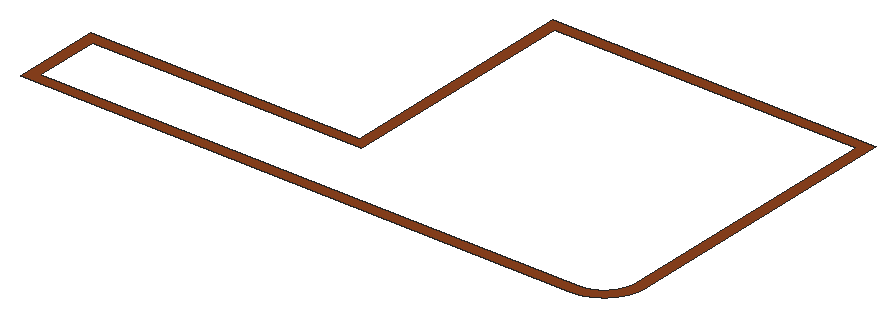
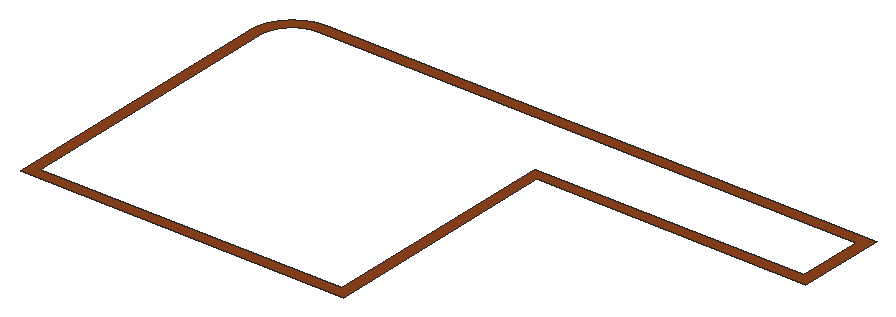
# SketchUp Ruby script. Lengths in inches.
U = 1.inch
M = Sketchup.active_model
def pt(a) = Geom::Point3d.new(a.map { |v| v * U })
def face(e, loops, mat)
  f = e.add_face(loops[0].map { |a| pt(a) })
  loops[1..].each { |l| e.add_face(l.map { |a| pt(a) }).erase! }
  f.material = f.back_material = mat if mat
  f
end
# faces: each face lists its corners as indices into pts; further lists are holes
def faces(e, pts, list, mat = nil) = list.each { |f| face(e, (f[0].is_a?(Array) ? f : [f]).map { |l| l.map { |i| pts[i] } }, mat) }
# xy, xz, yz: faces in a plane at the given z, y or x. An outline is a flat list of corners, or four numbers for a rectangle; further outlines are holes
def ring(l) = l.size == 4 ? [[l[0], l[1]], [l[2], l[1]], [l[2], l[3]], [l[0], l[3]]] : l.each_slice(2).to_a
def flat(e, list, mat, &to3) = list.each { |f| face(e, (f[0].is_a?(Array) ? f : [f]).map { |l| ring(l).map { |u, v| to3.(u, v) } }, mat) }
def xy(e, z, list, mat = nil) = flat(e, list, mat) { |x, y| [x, y, z] }
def xz(e, y, list, mat = nil) = flat(e, list, mat) { |x, z| [x, y, z] }
def yz(e, x, list, mat = nil) = flat(e, list, mat) { |y, z| [x, y, z] }
def lines(e, pts, list) = list.each { |a, b| e.add_line(pt(pts[a]), pt(pts[b])) }
# prism: a flat outline (further loops are holes) pulled along v
def prism(e, loops, v, mat = nil)
  f = face(e, loops, mat); d = Geom::Vector3d.new(v.map { |x| x * U })
  f.pushpull(f.normal.samedirection?(d) ? d.length : -d.length)
end
def box(e, o, s, mat = nil) = prism(e, [[o, [o[0] + s[0], o[1], o[2]], [o[0] + s[0], o[1] + s[1], o[2]], [o[0], o[1] + s[1], o[2]]]], [0, 0, s[2]], mat)
def at(x, y, z, deg = 0) = Geom::Transformation.translation(pt([x, y, z])) * Geom::Transformation.rotation(ORIGIN, Z_AXIS, deg.degrees)
def axes(o, x, y, z) = Geom::Transformation.new([*x, 0, *y, 0, *z, 0, *pt(o).to_a, 1])
def part(name) = M.definitions.add(name)
# library, detail: a bought-in or finely detailed component or shape, given as its bounding box
def library(name, o, s) = part(name).tap { |d| box(d.entities, o, s) }
def detail(e, o, s) = box(e.add_group.entities, o, s)
def put(e, d, t, mat = nil) = e.add_instance(d, t).tap { |i| i.material = mat if mat }
def group(e, t, mat = nil) = e.add_group.tap { |g| g.transformation = t; g.material = mat if mat }.entities
root = M.entities
M.materials.add("[Wood Fence]").color = [142, 67, 30]
xy(root,231,[[[24,164,24,212,171,212,171,344,348,344,348,187.6875,347.99,187.37,347.98,187.06,347.97,186.74,347.93,186.12,347.9,185.8,347.87,185.49,347.75,184.56,347.7,184.25,347.6,183.625,347.54,183.32,347.48,183.01,347.41,182.7,347.34,182.4,347.26,182.09,347.1,181.49,347.01,181.18,346.83,180.58,346.73,180.29,346.52,179.69,346.41,179.4,345.93,178.24,345.8,177.95,345.52,177.39,345.38,177.1,345.24,176.83,344.94,176.27,344.78,176,344.625,175.73,344.46,175.46,344.3,175.19,343.96,174.67,343.42,173.89,342.85,173.14,342.65,172.9,342.45,172.65,342.25,172.41,342.04,172.18,341.84,171.94,341.41,171.48,341.19,171.25,340.75,170.81,340.52,170.59,340.06,170.16,339.82,169.96,339.59,169.75,339.35,169.55,339.1,169.35,338.86,169.15,338.11,168.58,337.33,168.04,336.81,167.7,336.54,167.54,336.27,167.375,336,167.22,335.73,167.06,335.17,166.76,334.9,166.62,334.61,166.48,334.05,166.2,333.76,166.07,332.6,165.59,332.31,165.48,331.71,165.27,331.42,165.17,330.82,164.99,330.51,164.9,329.91,164.74,329.6,164.66,329.3,164.59,328.99,164.52,328.68,164.46,328.375,164.4,327.75,164.3,327.44,164.25,326.51,164.13,326.2,164.1,325.88,164.07,325.26,164.03,324.94,164.02,324.63,164.01,324.3125,164],[30,170,324.24,170,324.47,170.01,324.71,170.01,324.94,170.02,325.18,170.04,325.41,170.06,325.65,170.08,325.88,170.1,326.12,170.125,326.35,170.15,326.58,170.1875,326.82,170.22,327.28,170.3,327.51,170.35,327.74,170.39,327.97,170.44,328.2,170.5,328.43,170.55,328.66,170.61,328.89,170.68,329.11,170.74,329.34,170.81,329.5625,170.88,329.79,170.96,330.01,171.03,330.23,171.11,330.45,171.2,330.67,171.28,331.11,171.46,331.32,171.56,331.54,171.65,331.75,171.75,331.96,171.86,332.17,171.96,332.59,172.18,332.8,172.3,333,172.41,333.4,172.65,333.61,172.78,333.8,172.9,334,173.03,334.2,173.17,334.39,173.3,334.58,173.4375,334.77,173.58,334.96,173.72,335.14,173.86,335.33,174.01,335.51,174.16,335.69,174.3125,335.87,174.47,336.04,174.625,336.22,174.78,336.39,174.94,336.56,175.11,336.73,175.27,336.89,175.44,337.06,175.61,337.22,175.78,337.375,175.96,337.53,176.13,337.6875,176.31,337.84,176.49,337.99,176.67,338.14,176.86,338.28,177.04,338.42,177.23,338.5625,177.42,338.7,177.61,338.83,177.8,338.97,178,339.1,178.2,339.22,178.39,339.35,178.6,339.59,179,339.7,179.2,339.82,179.41,340.04,179.83,340.14,180.04,340.25,180.25,340.35,180.46,340.44,180.68,340.54,180.89,340.72,181.33,340.8,181.55,340.89,181.77,340.97,181.99,341.04,182.21,341.12,182.4375,341.19,182.66,341.26,182.89,341.32,183.11,341.39,183.34,341.45,183.57,341.5,183.8,341.56,184.03,341.61,184.26,341.65,184.49,341.7,184.72,341.78,185.18,341.8125,185.42,341.85,185.65,341.875,185.88,341.9,186.12,341.92,186.35,341.94,186.59,341.96,186.82,341.98,187.06,341.99,187.29,341.99,187.53,342,187.76,342,338,177,338,177,206,30,206]]],"[Wood Fence]")
